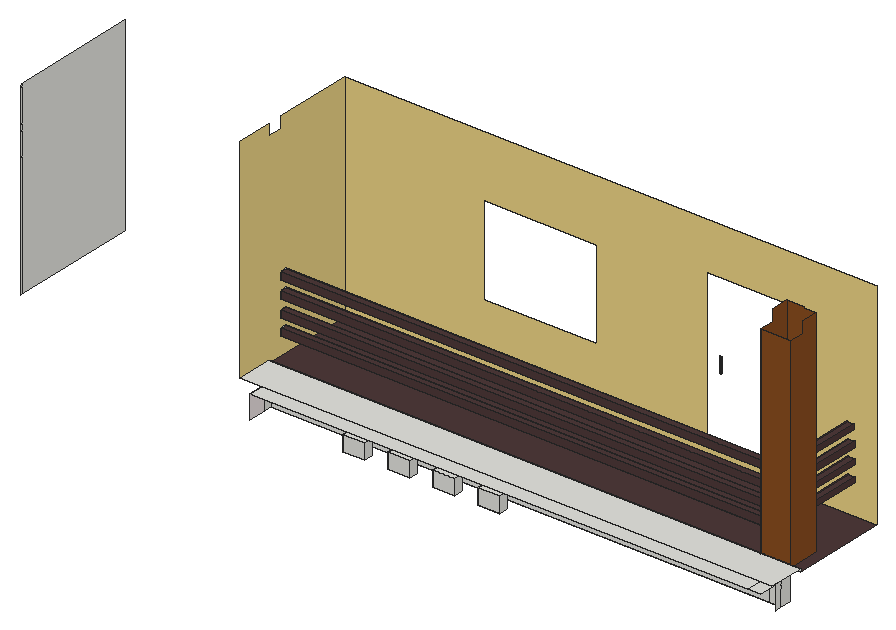
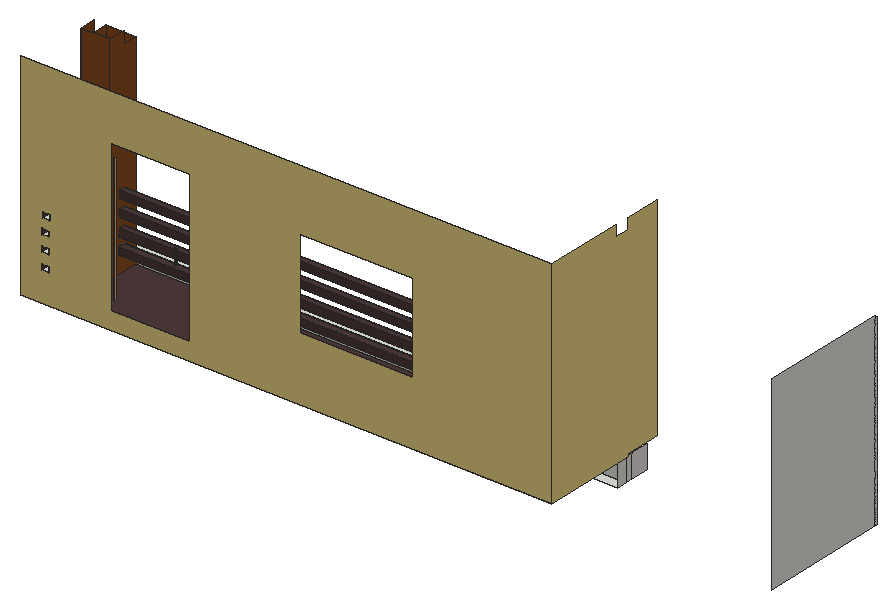
# SketchUp Ruby script. Lengths in inches.
U = 1.inch
M = Sketchup.active_model
def pt(a) = Geom::Point3d.new(a.map { |v| v * U })
def face(e, loops, mat)
  f = e.add_face(loops[0].map { |a| pt(a) })
  loops[1..].each { |l| e.add_face(l.map { |a| pt(a) }).erase! }
  f.material = f.back_material = mat if mat
  f
end
# faces: each face lists its corners as indices into pts; further lists are holes
def faces(e, pts, list, mat = nil) = list.each { |f| face(e, (f[0].is_a?(Array) ? f : [f]).map { |l| l.map { |i| pts[i] } }, mat) }
# xy, xz, yz: faces in a plane at the given z, y or x. An outline is a flat list of corners, or four numbers for a rectangle; further outlines are holes
def ring(l) = l.size == 4 ? [[l[0], l[1]], [l[2], l[1]], [l[2], l[3]], [l[0], l[3]]] : l.each_slice(2).to_a
def flat(e, list, mat, &to3) = list.each { |f| face(e, (f[0].is_a?(Array) ? f : [f]).map { |l| ring(l).map { |u, v| to3.(u, v) } }, mat) }
def xy(e, z, list, mat = nil) = flat(e, list, mat) { |x, y| [x, y, z] }
def xz(e, y, list, mat = nil) = flat(e, list, mat) { |x, z| [x, y, z] }
def yz(e, x, list, mat = nil) = flat(e, list, mat) { |y, z| [x, y, z] }
def lines(e, pts, list) = list.each { |a, b| e.add_line(pt(pts[a]), pt(pts[b])) }
# prism: a flat outline (further loops are holes) pulled along v
def prism(e, loops, v, mat = nil)
  f = face(e, loops, mat); d = Geom::Vector3d.new(v.map { |x| x * U })
  f.pushpull(f.normal.samedirection?(d) ? d.length : -d.length)
end
def box(e, o, s, mat = nil) = prism(e, [[o, [o[0] + s[0], o[1], o[2]], [o[0] + s[0], o[1] + s[1], o[2]], [o[0], o[1] + s[1], o[2]]]], [0, 0, s[2]], mat)
def at(x, y, z, deg = 0) = Geom::Transformation.translation(pt([x, y, z])) * Geom::Transformation.rotation(ORIGIN, Z_AXIS, deg.degrees)
def axes(o, x, y, z) = Geom::Transformation.new([*x, 0, *y, 0, *z, 0, *pt(o).to_a, 1])
def part(name) = M.definitions.add(name)
# library, detail: a bought-in or finely detailed component or shape, given as its bounding box
def library(name, o, s) = part(name).tap { |d| box(d.entities, o, s) }
def detail(e, o, s) = box(e.add_group.entities, o, s)
def put(e, d, t, mat = nil) = e.add_instance(d, t).tap { |i| i.material = mat if mat }
def group(e, t, mat = nil) = e.add_group.tap { |g| g.transformation = t; g.material = mat if mat }.entities
root = M.entities
M.materials.add("Generic").color = [136, 77, 32]
M.materials.add("Generic\#2").color = [78, 57, 57]
M.materials.add("Generic\#3").color = [235, 210, 133]
M.materials.add("Generic\#5").color = [232, 222, 222]
M.materials.add("Material \#1").color = [140, 140, 140]
c1 = library("3DGeom~9_Defintion",[456.52,-471.89,-18.89],[5.57,1000,5.49])
xy(root,122.7629,[[180.7096,46.9375,193.0221,51.9375],[205.9596,46.9375,218.2721,51.9375],[231.2096,46.9375,243.5221,51.9375],[256.4596,46.9375,268.7721,51.9375]])
xy(root,131.3879,[[180.7096,46.9375,193.0221,51.9375],[205.9596,46.9375,218.2721,51.9375],[231.2096,46.9375,243.5221,51.9375],[256.4596,46.9375,268.7721,51.9375]])
xy(root,137.6106,[[411.67,41.4375,418.8848,51.9375],[411.67,51.9375,418.8848,55.875]])
xy(root,141.9375,[[412.79,61.6875,419.4775,79.5282]])
xy(root,141.9375,[[127.5829,61.6875,127.5829,114.8125,424.8848,114.8125,424.8848,61.6875,419.4775,61.6875,419.4775,79.5282,402.9775,79.5282,402.9775,61.6875]],"Generic\#2")
xy(root,143.5,[[127.5829,41.4375,424.8848,61.6875]])
xy(root,158.7077,[[409.2127,79.5282,412.7127,114.8126]])
xy(root,161.8952,[[409.2127,79.5282,412.7127,114.8126]],"Generic\#2")
xy(root,167.7702,[[409.2127,79.5282,412.7127,114.8126]])
xy(root,170.9577,[[409.2127,79.5282,412.7127,114.8126]],"Generic\#2")
xy(root,176.5202,[[409.2127,79.5282,412.7127,114.8126]])
xy(root,179.7077,[[409.2127,79.5282,412.7127,114.8126]],"Generic\#2")
xy(root,184.9607,[[408.521,79.5282,412.021,114.8126]])
xy(root,188.1482,[[408.521,79.5282,412.021,114.8126]],"Generic\#2")
xy(root,190.2391,[[338.0444,114.5846,338.0444,114.9056,338.0796,114.9056],[338.0444,114.5846,338.0796,114.9056,338.0796,114.5846]],"Material \#1")
xy(root,190.5551,[[338.0267,114.5846,338.0855,114.5846,338.0267,114.9056],[338.0855,114.5846,338.0855,114.9056,338.0267,114.9056]],"Material \#1")
xz(root,46.9375,[[180.7096,122.7629,193.0221,131.3879],[205.9596,122.7629,218.2721,131.3879],[231.2096,122.7629,243.5221,131.3879],[256.4596,122.7629,268.7721,131.3879]])
xz(root,55.875,[[411.67,124.5524,411.67,137.6106,133.3329,137.6107,133.334,124.5525],[411.67,124.5524,418.8844,124.5524,418.8848,137.6106,411.67,137.6106]])
xz(root,61.6875,[[127.5829,141.9375,402.9775,143.5],[402.9775,141.9375,412.79,143.5],[412.79,141.9375,419.4775,143.5],[419.4775,141.9375,424.8848,143.5]])
xz(root,61.6875,[[402.9775,143.5,419.4775,255.6875]],"Generic")
xz(root,69.8538,[[127.5793,151.8312,402.9775,155.8937],[127.5793,160.9562,402.9775,165.0187],[127.5793,170.6437,402.9775,174.7062],[127.5793,180.1437,402.9775,184.2062]],"Generic\#2")
xz(root,73.6426,[[127.5793,151.8384,402.9775,155.9009],[127.5793,160.9634,402.9775,165.0259],[127.5793,170.6509,402.9775,174.7134],[127.5793,180.1509,402.9775,184.2134]],"Generic\#2")
xz(root,79.5282,[[409.2127,158.7077,412.7127,161.8952],[409.2127,167.7702,412.7127,170.9577],[409.2127,176.5202,412.7127,179.7077],[408.521,184.9607,412.021,188.1482]])
xz(root,79.5282,[[[402.9775,141.9375,419.4775,141.9375,419.4775,261.9375,412.79,261.9375,412.79,262.375,402.9775,262.375],[408.521,184.9607,412.021,188.1482],[409.2127,176.5202,412.7127,179.7077],[409.2127,167.7702,412.7127,170.9577],[409.2127,158.7077,412.7127,161.8952]]],"Generic")
xz(root,114.5846,[[338.0558,190.1859,337.9996,190.1931,338.0558,190.1938],[338.0558,190.1859,338.0558,190.1938,338.1099,190.2008],[338.0558,190.1859,338.1099,190.2008,338.1121,190.1931],[337.9996,190.1931,337.9472,190.2142,338.0017,190.2008],[337.9996,190.1931,338.0017,190.2008,338.0558,190.1938],
  [338.1121,190.1931,338.1099,190.2008,338.1603,190.2211],[338.1121,190.1931,338.1603,190.2211,338.1644,190.2142],[338.0017,190.2008,337.9472,190.2142,337.9513,190.2211],[337.9472,190.2142,337.9023,190.2477,337.9513,190.2211],[338.1644,190.2142,338.1603,190.2211,338.2036,190.2534],
  [338.1644,190.2142,338.2036,190.2534,338.2094,190.2477],[337.9513,190.2211,337.9023,190.2477,337.9081,190.2534],[337.9023,190.2477,337.8677,190.2915,337.9081,190.2534],[338.2094,190.2477,338.2036,190.2534,338.2369,190.2955],[338.2094,190.2477,338.2369,190.2955,338.2439,190.2915],
  [337.9081,190.2534,337.8677,190.2915,337.8748,190.2955],[337.8677,190.2915,337.846,190.3424,337.8748,190.2955],[338.2439,190.2915,338.2369,190.2955,338.2577,190.3445],[338.2439,190.2915,338.2577,190.3445,338.2656,190.3424],[337.8748,190.2955,337.846,190.3424,337.854,190.3445],
  [337.846,190.3424,337.8386,190.3971,337.854,190.3445],[338.2656,190.3424,338.2577,190.3445,338.2649,190.3971],[338.2656,190.3424,338.2649,190.3971,338.273,190.3971],[337.854,190.3445,337.8386,190.3971,337.8468,190.3971],[337.8386,190.3971,337.846,190.4517,337.8468,190.3971],
  [337.8468,190.3971,337.846,190.4517,337.854,190.4497],[338.2649,190.3971,338.2577,190.4497,338.273,190.3971],[338.273,190.3971,338.2577,190.4497,338.2656,190.4517],[337.854,190.4497,337.846,190.4517,337.8677,190.5027],[337.854,190.4497,337.8677,190.5027,337.8748,190.4987],
  [338.2577,190.4497,338.2369,190.4987,338.2656,190.4517],[338.2656,190.4517,338.2369,190.4987,338.2439,190.5027],[337.8748,190.4987,337.8677,190.5027,337.9023,190.5464],[337.8748,190.4987,337.9023,190.5464,337.9081,190.5408],[338.2369,190.4987,338.2036,190.5408,338.2439,190.5027],
  [338.2439,190.5027,338.2036,190.5408,338.2094,190.5464],[337.9081,190.5408,337.9023,190.5464,337.9472,190.58],[337.9081,190.5408,337.9472,190.58,337.9513,190.5731],[338.2036,190.5408,338.1603,190.5731,338.2094,190.5464],[338.2094,190.5464,338.1603,190.5731,338.1644,190.58],
  [337.9513,190.5731,337.9472,190.58,337.9996,190.6011],[337.9513,190.5731,337.9996,190.6011,338.0017,190.5934],[338.1603,190.5731,338.1099,190.5934,338.1644,190.58],[338.1644,190.58,338.1099,190.5934,338.1121,190.6011],[338.0017,190.5934,337.9996,190.6011,338.0558,190.6083],
  [338.0017,190.5934,338.0558,190.6083,338.0558,190.6003],[338.1099,190.5934,338.0558,190.6003,338.1121,190.6011],[338.0558,190.6003,338.0558,190.6083,338.1121,190.6011]],"Material \#1")
xz(root,114.595,[[338.0558,189.7138,337.9354,189.77,338.1763,189.77],[338.0558,189.7138,337.988,189.729,337.9354,189.77],[338.0558,189.7138,338.0205,189.7177,337.988,189.729],[338.0558,189.7138,338.1237,189.729,338.0912,189.7177],[338.0558,189.7138,338.1763,189.77,338.1237,189.729],
  [337.988,189.729,337.9593,189.7468,337.9354,189.77],[338.1237,189.729,338.1763,189.77,338.1523,189.7468],[338.1763,189.77,337.782,190.3616,337.8657,190.2489],[338.1763,189.77,337.8956,190.1739,337.782,190.3616],[338.1763,189.77,337.8657,190.2489,337.9035,190.2122],
  [338.1763,189.77,337.8982,190.1686,337.8956,190.1739],[338.1763,189.77,337.9,190.163,337.8982,190.1686],[338.1763,189.77,337.9011,190.1571,337.9,190.163],[337.9354,189.77,337.9011,190.1571,338.1763,189.77],[337.9354,189.77,337.9015,190.151,337.9011,190.1571],
  [337.9354,189.77,337.9056,189.8295,337.9015,190.151],[338.1763,189.77,337.9035,190.2122,337.9487,190.1842],[337.9354,189.77,337.9172,189.7979,337.9056,189.8295],[338.1763,189.77,337.9487,190.1842,338,190.1664],[338.1763,189.77,338,190.1664,338.0558,190.1601],
  [338.1763,189.77,338.0558,190.1601,338.2102,189.8639],[338.1763,189.77,338.2061,189.8295,338.1945,189.7979],[338.1763,189.77,338.2102,189.8639,338.2061,189.8295],[337.9056,189.8295,337.9015,189.8639,337.9015,190.151],[338.2102,189.8639,338.0558,190.1601,338.1117,190.1664],
  [338.2102,189.8639,338.1117,190.1664,338.163,190.1842],[338.2102,189.8639,338.163,190.1842,338.2082,190.2122],[338.2102,189.8639,338.2082,190.2122,338.2102,190.151],[338.2102,190.151,338.2082,190.2122,338.2118,190.1636],[338.2102,190.151,338.2118,190.1636,338.2106,190.1576],
  [338.2118,190.1636,338.2082,190.2122,338.246,190.2489],[338.2118,190.1636,338.2165,190.1744,338.2137,190.1692],[338.2118,190.1636,338.246,190.2489,338.2165,190.1744],[337.8956,190.1739,337.8921,190.179,337.782,190.3616],[338.2165,190.1744,338.246,190.2489,338.2748,190.2929],
  [338.2165,190.1744,338.2748,190.2929,338.3295,190.3617],[338.2165,190.1744,338.3295,190.3617,338.2199,190.1792],[337.8921,190.179,337.8877,190.1839,337.782,190.3616],[338.2199,190.1792,338.3295,190.3617,338.2241,190.1839],[337.8877,190.1839,337.8346,190.2365,337.782,190.3616],
  [337.8877,190.1839,337.8825,190.1885,337.8346,190.2365],[338.2241,190.1839,338.2761,190.2374,338.229,190.1883],[338.2241,190.1839,338.3295,190.3617,338.2761,190.2374],[338.229,190.1883,338.2761,190.2374,338.2539,190.2116],[337.8825,190.1885,337.857,190.2111,337.8346,190.2365],
  [337.8346,190.2365,337.8004,190.295,337.782,190.3616],[337.8346,190.2365,337.8156,190.2646,337.8004,190.295],[338.2761,190.2374,338.3107,190.2957,338.2952,190.2655],[338.2761,190.2374,338.3295,190.3617,338.3107,190.2957],[337.8657,190.2489,337.782,190.3616,337.8369,190.2929],
  [337.8369,190.2929,337.782,190.3616,337.8186,190.3428],[338.2748,190.2929,338.2931,190.3428,338.3295,190.3617],[337.8004,190.295,337.789,190.3274,337.782,190.3616],[338.3107,190.2957,338.3295,190.3617,338.3223,190.3278],[337.8186,190.3428,337.782,190.3616,337.8121,190.3971],
  [338.2931,190.3428,338.2995,190.3971,338.3295,190.3617],[337.782,190.3616,337.7796,190.3971,337.7869,190.4586],[337.782,190.3616,337.7869,190.4586,337.8404,190.565],[337.782,190.3616,337.8186,190.4514,337.8121,190.3971],[337.782,190.3616,337.8404,190.565,337.8186,190.4514],
  [338.3295,190.3617,338.2713,190.565,338.3247,190.4586],[338.3295,190.3617,338.2748,190.5012,338.2713,190.565],[338.3295,190.3617,338.2931,190.4514,338.2748,190.5012],[338.3295,190.3617,338.2995,190.3971,338.2931,190.4514],[338.3295,190.3617,338.3247,190.4586,338.332,190.3971],
  [337.8186,190.4514,337.8404,190.565,337.8369,190.5012],[337.7869,190.4586,337.8077,190.5151,337.8404,190.565],[338.3247,190.4586,338.2713,190.565,338.3039,190.5151],[337.8369,190.5012,337.8404,190.565,337.8657,190.5453],[338.2748,190.5012,338.246,190.5453,338.2713,190.565],
  [337.8657,190.5453,337.8404,190.565,337.9035,190.582],[338.246,190.5453,338.2082,190.582,338.2713,190.565],[337.8404,190.565,337.8832,190.6066,337.9344,190.6383],[337.8404,190.565,337.9344,190.6383,338.0558,190.6657],[337.8404,190.565,337.9487,190.61,337.9035,190.582],
  [337.8404,190.565,338.0558,190.6657,337.9487,190.61],[338.2713,190.565,338.0558,190.6657,338.1772,190.6383],[338.2713,190.565,338.163,190.61,338.0558,190.6657],[338.2713,190.565,338.2082,190.582,338.163,190.61],[338.2713,190.565,338.1772,190.6383,338.2285,190.6066],
  [337.9487,190.61,338.0558,190.6657,338,190.6278],[338.163,190.61,338.1117,190.6278,338.0558,190.6657],[338,190.6278,338.0558,190.6657,338.0558,190.6341],[338.1117,190.6278,338.0558,190.6341,338.0558,190.6657],[337.9344,190.6383,337.9926,190.6586,338.0558,190.6657],
  [338.1772,190.6383,338.0558,190.6657,338.1191,190.6586]],"Material \#1")
xz(root,114.6295,[[338.0558,187.3364,337.9281,187.3476,338.0558,187.3483],[338.0558,187.3364,338.0558,187.3483,338.1814,187.3593],[338.0558,187.3364,338.1814,187.3593,338.1836,187.3476],[337.9281,187.3476,337.8081,187.3796,337.9303,187.3593],[337.9281,187.3476,337.9303,187.3593,338.0558,187.3483],
  [338.1836,187.3476,338.1814,187.3593,338.2993,187.3908],[338.1836,187.3476,338.2993,187.3908,338.3036,187.3796],[337.9303,187.3593,337.8081,187.3796,337.8123,187.3908],[337.8081,187.3796,337.6975,187.4307,337.8123,187.3908],[338.3036,187.3796,338.2993,187.3908,338.408,187.441],
  [338.3036,187.3796,338.408,187.441,338.4142,187.4307],[337.8123,187.3908,337.6975,187.4307,337.7037,187.441],[337.6975,187.4307,337.5983,187.499,337.7037,187.441],[338.4142,187.4307,338.408,187.441,338.5055,187.508],[338.4142,187.4307,338.5055,187.508,338.5134,187.499],
  [337.7037,187.441,337.5983,187.499,337.6062,187.508],[337.5983,187.499,337.5126,187.5823,337.6062,187.508],[338.5134,187.499,338.5055,187.508,338.5897,187.59],[338.5134,187.499,338.5897,187.59,338.5991,187.5823],[337.6062,187.508,337.5126,187.5823,337.5219,187.59],
  [338.0558,187.5212,338.0136,187.5249,338.0558,187.5331],[338.0558,187.5212,338.0558,187.5331,338.0959,187.5366],[338.0558,187.5212,338.0959,187.5366,338.0981,187.5249],[338.0136,187.5249,337.9736,187.5356,338.0158,187.5366],[338.0136,187.5249,338.0158,187.5366,338.0558,187.5331],
  [338.0981,187.5249,338.0959,187.5366,338.1339,187.5468],[338.0981,187.5249,338.1339,187.5468,338.1381,187.5356],[337.9736,187.5356,337.9367,187.5526,337.9778,187.5468],[337.9736,187.5356,337.9778,187.5468,338.0158,187.5366],[338.1381,187.5356,338.1339,187.5468,338.1688,187.5629],
  [338.1381,187.5356,338.1688,187.5629,338.175,187.5526],[337.9778,187.5468,337.9367,187.5526,337.9429,187.5629],[337.9367,187.5526,337.9038,187.5753,337.9429,187.5629],[338.175,187.5526,338.1688,187.5629,338.2,187.5844],[338.175,187.5526,338.2,187.5844,338.2079,187.5753],
  [337.9429,187.5629,337.9038,187.5753,337.9117,187.5844],[337.9038,187.5753,337.8754,187.6029,337.9117,187.5844],[338.2079,187.5753,338.2,187.5844,338.2269,187.6105],[338.2079,187.5753,338.2269,187.6105,338.2363,187.6029],[337.5126,187.5823,337.446,187.6728,337.5219,187.59],
  [338.5991,187.5823,338.5897,187.59,338.6587,187.6848],[338.5991,187.5823,338.6587,187.6848,338.6692,187.6788],[337.9117,187.5844,337.8754,187.6029,337.8848,187.6105],[337.5219,187.59,337.446,187.6728,337.4566,187.6789],[337.8754,187.6029,337.8521,187.6349,337.8848,187.6105],
  [338.2363,187.6029,338.2269,187.6105,338.249,187.6409],[338.2363,187.6029,338.249,187.6409,338.2596,187.6349],[337.8848,187.6105,337.8521,187.6349,337.8627,187.6409],[337.8521,187.6349,337.8346,187.6707,337.8627,187.6409],[338.2596,187.6349,338.249,187.6409,338.2656,187.6749],
  [338.2596,187.6349,338.2656,187.6749,338.2771,187.6707],[337.8627,187.6409,337.8346,187.6707,337.8461,187.6749],[337.8346,187.6707,337.8236,187.7096,337.8461,187.6749],[338.2771,187.6707,338.2656,187.6749,338.2761,187.7118],[338.2771,187.6707,338.2761,187.7118,338.2881,187.7097],
  [337.446,187.6728,337.3899,187.7863,337.4566,187.6789],[337.8461,187.6749,337.8236,187.7096,337.8356,187.7118],[338.6692,187.6788,338.6587,187.6848,338.7103,187.7904],[338.6692,187.6788,338.7103,187.7904,338.7218,187.7863],[337.4566,187.6789,337.3899,187.7863,337.4014,187.7905],
  [337.8236,187.7096,337.8198,187.7467,337.8356,187.7118],[338.2881,187.7097,338.2761,187.7118,338.2796,187.7507],[338.2881,187.7097,338.2796,187.7507,338.2919,187.7507],[337.8356,187.7118,337.8198,187.7467,337.832,187.7468],[337.8198,187.7467,337.8236,187.7917,337.832,187.7468],
  [337.832,187.7468,337.8236,187.7917,337.8356,187.7897],[338.2796,187.7507,338.2761,187.7897,338.2919,187.7507],[338.2919,187.7507,338.2761,187.7897,338.2881,187.7918],[337.3899,187.7863,337.3569,187.903,337.4014,187.7905],[338.7218,187.7863,338.7103,187.7904,338.7427,187.9051],
  [338.7218,187.7863,338.7427,187.9051,338.7548,187.903],[337.8356,187.7897,337.8236,187.7917,337.8346,187.8308],[337.8356,187.7897,337.8346,187.8308,337.8461,187.8266],[338.2761,187.7897,338.2656,187.8266,338.2881,187.7918],[337.4014,187.7905,337.3569,187.903,337.369,187.9051],
  [338.2881,187.7918,338.2656,187.8266,338.2771,187.8308],[337.8461,187.8266,337.8346,187.8308,337.8521,187.8666],[337.8461,187.8266,337.8521,187.8666,337.8627,187.8606],[338.2656,187.8266,338.249,187.8606,338.2771,187.8308],[338.2771,187.8308,338.249,187.8606,338.2596,187.8666],
  [337.8627,187.8606,337.8521,187.8666,337.8754,187.8986],[337.8627,187.8606,337.8754,187.8986,337.8848,187.8909],[338.249,187.8606,338.2269,187.8909,338.2596,187.8666],[338.2596,187.8666,338.2269,187.8909,338.2363,187.8986],[337.8848,187.8909,337.8754,187.8986,337.9038,187.9262],
  [337.8848,187.8909,337.9038,187.9262,337.9117,187.9171],[338.2269,187.8909,338.2,187.9171,338.2363,187.8986],[338.2363,187.8986,338.2,187.9171,338.2079,187.9262],[337.3569,187.903,337.345,188.0316,337.369,187.9051],[338.7548,187.903,338.7427,187.9051,338.7545,188.0322],
  [338.7548,187.903,338.7545,188.0322,338.7666,188.0316],[337.369,187.9051,337.345,188.0316,337.3572,188.0322],[337.9117,187.9171,337.9038,187.9262,337.9367,187.9488],[337.9117,187.9171,337.9367,187.9488,337.9429,187.9386],[338.2,187.9171,338.1688,187.9386,338.2079,187.9262],
  [338.2079,187.9262,338.1688,187.9386,338.175,187.9488],[337.9429,187.9386,337.9367,187.9488,337.9736,187.9659],[337.9429,187.9386,337.9736,187.9659,337.9778,187.9547],[338.1688,187.9386,338.1339,187.9547,338.175,187.9488],[338.175,187.9488,338.1339,187.9547,338.1381,187.9659],
  [337.9778,187.9547,337.9736,187.9659,338.0136,187.9766],[337.9778,187.9547,338.0136,187.9766,338.0158,187.9649],[338.1339,187.9547,338.0959,187.9649,338.1381,187.9659],[338.0158,187.9649,338.0136,187.9766,338.0558,187.9803],[338.0158,187.9649,338.0558,187.9803,338.0558,187.9684],
  [338.0959,187.9649,338.0558,187.9684,338.0981,187.9766],[338.0959,187.9649,338.0981,187.9766,338.1381,187.9659],[338.0558,187.9684,338.0558,187.9803,338.0981,187.9766],[337.345,188.0316,337.345,195.9223,337.3572,188.0322],[338.7666,188.0316,338.7545,188.0322,338.7545,194.2213],
  [338.7666,188.0316,338.7545,194.2213,338.7545,195.9218],[338.7666,188.0316,338.7545,195.9218,338.7666,195.9223],[337.3572,188.0322,337.345,195.9223,337.3572,195.9218]],"Material \#1")
xz(root,114.664,[[338.0558,190.1601,337.9928,190.1682,338.0558,190.1681],[338.0558,190.1601,338.0558,190.1681,338.1168,190.1759],[338.0558,190.1601,338.1168,190.1759,338.1189,190.1682],[338.0558,190.1681,337.9928,190.1682,337.9949,190.1759],[337.9928,190.1682,337.934,190.1918,337.9949,190.1759],
  [338.1189,190.1682,338.1168,190.1759,338.1736,190.1987],[338.1189,190.1682,338.1736,190.1987,338.1777,190.1918],[337.9949,190.1759,337.934,190.1918,337.9381,190.1987],[337.934,190.1918,337.8835,190.2295,337.9381,190.1987],[338.1777,190.1918,338.1736,190.1987,338.2224,190.2351],
  [338.1777,190.1918,338.2224,190.2351,338.2282,190.2295],[337.9381,190.1987,337.8835,190.2295,337.8893,190.2351],[337.8835,190.2295,337.8448,190.2786,337.8893,190.2351],[338.2282,190.2295,338.2224,190.2351,338.2598,190.2826],[338.2282,190.2295,338.2598,190.2826,338.2669,190.2786],
  [337.8893,190.2351,337.8448,190.2786,337.8519,190.2826],[337.8448,190.2786,337.8204,190.3357,337.8519,190.2826],[338.2669,190.2786,338.2598,190.2826,338.2833,190.3378],[338.2669,190.2786,338.2833,190.3378,338.2912,190.3357],[337.8519,190.2826,337.8204,190.3357,337.8284,190.3378],
  [337.8204,190.3357,337.8121,190.3971,337.8284,190.3378],[338.2912,190.3357,338.2833,190.3378,338.2914,190.3971],[338.2912,190.3357,338.2914,190.3971,338.2995,190.3971],[337.8284,190.3378,337.8121,190.3971,337.8203,190.3971],[337.8121,190.3971,337.8204,190.4584,337.8203,190.3971],
  [337.8203,190.3971,337.8204,190.4584,337.8284,190.4564],[338.2914,190.3971,338.2833,190.4564,338.2995,190.3971],[338.2995,190.3971,338.2833,190.4564,338.2912,190.4584],[337.8284,190.4564,337.8204,190.4584,337.8448,190.5156],[337.8284,190.4564,337.8448,190.5156,337.8519,190.5116],
  [338.2833,190.4564,338.2598,190.5116,338.2912,190.4584],[338.2912,190.4584,338.2598,190.5116,338.2669,190.5156],[337.8519,190.5116,337.8448,190.5156,337.8835,190.5647],[337.8519,190.5116,337.8835,190.5647,337.8893,190.559],[338.2598,190.5116,338.2224,190.559,338.2669,190.5156],
  [338.2669,190.5156,338.2224,190.559,338.2282,190.5647],[337.8893,190.559,337.8835,190.5647,337.934,190.6023],[337.8893,190.559,337.934,190.6023,337.9381,190.5954],[338.2224,190.559,338.1736,190.5954,338.2282,190.5647],[338.2282,190.5647,338.1736,190.5954,338.1777,190.6023],
  [337.9381,190.5954,337.934,190.6023,337.9928,190.626],[337.9381,190.5954,337.9928,190.626,337.9949,190.6183],[338.1736,190.5954,338.1168,190.6183,338.1777,190.6023],[338.1777,190.6023,338.1168,190.6183,338.1189,190.626],[337.9949,190.6183,337.9928,190.626,338.0558,190.6341],
  [337.9949,190.6183,338.0558,190.6341,338.0558,190.6261],[338.1168,190.6183,338.0558,190.6261,338.1189,190.626],[338.1189,190.626,338.0558,190.6261,338.0558,190.6341]],"Material \#1")
xz(root,114.8125,[[4.8848,141.9375,4.892,141.9375,4.8848,247.422]])
xz(root,114.9056,[[338.0444,190.2391,338.0326,190.2628,338.0679,190.2628],[338.0444,190.2391,338.0679,190.2628,338.0796,190.2391],[338.0326,190.2628,338.0264,190.2707,338.0741,190.2707],[338.0326,190.2628,338.0741,190.2707,338.0679,190.2628],[338.0264,190.2707,338.0264,190.2884,338.0741,190.2884],
  [338.0264,190.2707,338.0741,190.2884,338.0741,190.2707],[338.0264,190.2884,338.0326,190.2964,338.0679,190.2964],[338.0264,190.2884,338.0679,190.2964,338.0741,190.2884],[338.0326,190.2964,338.0326,190.326,338.0796,190.326],[338.0326,190.2964,338.0796,190.326,338.0679,190.2964],
  [338.0326,190.326,338.0326,190.3536,338.0796,190.3536],[338.0326,190.326,338.0796,190.3536,338.0796,190.326],[338.0326,190.3536,338.0237,190.376,338.0886,190.376],[338.0326,190.3536,338.0886,190.376,338.0796,190.3536],[338.0237,190.376,338.0237,190.3984,338.0886,190.3984],
  [338.0237,190.376,338.0886,190.3984,338.0886,190.376],[338.0237,190.3984,338.0326,190.4208,338.0796,190.4208],[338.0237,190.3984,338.0796,190.4208,338.0886,190.3984],[338.0326,190.4208,338.0267,190.4366,338.0855,190.4366],[338.0326,190.4208,338.0855,190.4366,338.0796,190.4208],
  [338.0267,190.4366,338.0267,190.4879,338.0855,190.4879],[338.0267,190.4366,338.0855,190.4879,338.0855,190.4366],[338.0267,190.4879,338.0339,190.4919,338.0783,190.4919],[338.0267,190.4879,338.0783,190.4919,338.0855,190.4879],[338.0339,190.4919,338.0339,190.4998,338.0783,190.4998],
  [338.0339,190.4919,338.0783,190.4998,338.0783,190.4919],[338.0339,190.4998,338.0267,190.5037,338.0855,190.5037],[338.0339,190.4998,338.0855,190.5037,338.0783,190.4998],[338.0267,190.5037,338.0267,190.5551,338.0855,190.5551],[338.0267,190.5037,338.0855,190.5551,338.0855,190.5037]],"Material \#1")
xz(root,114.9401,[[338.0558,189.7138,337.988,189.729,338.0205,189.7177],[338.0558,189.7138,338.1237,189.729,337.988,189.729],[338.0558,189.7138,338.0912,189.7177,338.1237,189.729],[337.988,189.729,337.9015,190.151,337.9056,189.8295],[337.988,189.729,338.2061,189.8295,337.9015,190.151],
  [337.988,189.729,337.9056,189.8295,337.9354,189.77],[337.988,189.729,337.9354,189.77,337.9593,189.7468],[337.988,189.729,338.1237,189.729,338.2061,189.8295],[338.1237,189.729,338.1523,189.7468,338.1763,189.77],[338.1237,189.729,338.1763,189.77,338.2061,189.8295],
  [337.9354,189.77,337.9056,189.8295,337.9172,189.7979],[338.1763,189.77,338.1945,189.7979,338.2061,189.8295],[338.2061,189.8295,337.8956,190.1739,337.8982,190.1686],[338.2061,189.8295,338.2102,189.8639,337.8956,190.1739],[338.2061,189.8295,337.8982,190.1686,337.9,190.163],
  [338.2061,189.8295,337.9,190.163,337.9011,190.1571],[338.2061,189.8295,337.9011,190.1571,337.9015,190.151],[337.9056,189.8295,337.9015,190.151,337.9015,189.8639],[338.2102,189.8639,337.8657,190.2489,337.8956,190.1739],[338.2102,189.8639,337.9035,190.2122,337.8657,190.2489],
  [338.2102,189.8639,337.9487,190.1842,337.9035,190.2122],[338.2102,189.8639,338,190.1664,337.9487,190.1842],[338.2102,189.8639,338.0558,190.1601,338,190.1664],[338.2102,189.8639,338.1117,190.1664,338.0558,190.1601],[338.2102,189.8639,338.2102,190.151,338.1117,190.1664],
  [338.2102,190.151,338.2118,190.1636,338.1117,190.1664],[338.2102,190.151,338.2106,190.1576,338.2118,190.1636],[338.2118,190.1636,338.2165,190.1744,338.1117,190.1664],[338.2118,190.1636,338.2137,190.1692,338.2165,190.1744],[338.1117,190.1664,338.2165,190.1744,338.163,190.1842],
  [337.8956,190.1739,337.782,190.3616,337.8921,190.179],[337.8956,190.1739,337.8369,190.2929,337.782,190.3616],[337.8956,190.1739,337.8657,190.2489,337.8369,190.2929],[338.2165,190.1744,338.2082,190.2122,338.163,190.1842],[338.2165,190.1744,338.246,190.2489,338.2082,190.2122],
  [338.2165,190.1744,338.2199,190.1792,338.3295,190.3617],[338.2165,190.1744,338.3295,190.3617,338.246,190.2489],[337.8921,190.179,337.782,190.3616,337.8877,190.1839],[338.2199,190.1792,338.2241,190.1839,338.3295,190.3617],[337.8877,190.1839,337.782,190.3616,337.8346,190.2365],
  [337.8877,190.1839,337.8346,190.2365,337.8825,190.1885],[338.2241,190.1839,338.229,190.1883,338.2761,190.2374],[338.2241,190.1839,338.2761,190.2374,338.3295,190.3617],[338.229,190.1883,338.2539,190.2116,338.2761,190.2374],[337.8825,190.1885,337.8346,190.2365,337.857,190.2111],
  [337.8346,190.2365,337.782,190.3616,337.8004,190.295],[337.8346,190.2365,337.8004,190.295,337.8156,190.2646],[338.2761,190.2374,338.2952,190.2655,338.3107,190.2957],[338.2761,190.2374,338.3107,190.2957,338.3295,190.3617],[338.246,190.2489,338.3295,190.3617,338.2748,190.2929],
  [337.8369,190.2929,337.8186,190.3428,337.782,190.3616],[338.2748,190.2929,338.3295,190.3617,338.2931,190.3428],[337.8004,190.295,337.782,190.3616,337.789,190.3274],[338.3107,190.2957,338.3223,190.3278,338.3295,190.3617],[337.8186,190.3428,337.8121,190.3971,337.782,190.3616],
  [338.2931,190.3428,338.3295,190.3617,338.2995,190.3971],[337.782,190.3616,337.7869,190.4586,337.7796,190.3971],[337.782,190.3616,337.8121,190.3971,337.8186,190.4514],[337.782,190.3616,337.8186,190.4514,337.8369,190.5012],[337.782,190.3616,337.8369,190.5012,337.8404,190.565],
  [337.782,190.3616,337.8404,190.565,337.7869,190.4586],[338.3295,190.3617,338.2713,190.565,338.2931,190.4514],[338.3295,190.3617,338.3247,190.4586,338.2713,190.565],[338.3295,190.3617,338.2931,190.4514,338.2995,190.3971],[338.3295,190.3617,338.332,190.3971,338.3247,190.4586],
  [338.2931,190.4514,338.2713,190.565,338.2748,190.5012],[337.7869,190.4586,337.8404,190.565,337.8077,190.5151],[338.3247,190.4586,338.3039,190.5151,338.2713,190.565],[337.8369,190.5012,337.8657,190.5453,337.8404,190.565],[338.2748,190.5012,338.2713,190.565,338.246,190.5453],
  [337.8657,190.5453,337.9035,190.582,337.8404,190.565],[338.246,190.5453,338.2713,190.565,338.2082,190.582],[337.8404,190.565,337.9035,190.582,337.9487,190.61],[337.8404,190.565,337.9344,190.6383,337.8832,190.6066],[337.8404,190.565,337.9487,190.61,338.0558,190.6657],
  [337.8404,190.565,338.0558,190.6657,337.9344,190.6383],[338.2713,190.565,338.0558,190.6657,338.163,190.61],[338.2713,190.565,338.1772,190.6383,338.0558,190.6657],[338.2713,190.565,338.163,190.61,338.2082,190.582],[338.2713,190.565,338.2285,190.6066,338.1772,190.6383],
  [337.9487,190.61,338,190.6278,338.0558,190.6657],[338.163,190.61,338.0558,190.6657,338.1117,190.6278],[338,190.6278,338.0558,190.6341,338.0558,190.6657],[338.1117,190.6278,338.0558,190.6657,338.0558,190.6341],[337.9344,190.6383,338.0558,190.6657,337.9926,190.6586],
  [338.1772,190.6383,338.1191,190.6586,338.0558,190.6657]],"Material \#1")
yz(root,4.8848,[[41.4375,141.9375,42.5,246.5106],[42.5,141.9375,114.8125,247.422]])
yz(root,127.5793,[[69.8538,151.8312,69.8538,155.8937,73.6426,155.9009,73.6426,151.8384],[69.8538,160.9562,69.8538,165.0187,73.6426,165.0259,73.6426,160.9634],[69.8538,170.6437,69.8538,174.7062,73.6426,174.7134,73.6426,170.6509],[69.8538,180.1437,69.8538,184.2062,73.6426,184.2134,73.6426,180.1509]])
yz(root,180.7096,[[46.9375,122.7629,51.9375,131.3879]])
yz(root,193.0221,[[46.9375,122.7629,51.9375,131.3879]])
yz(root,205.9596,[[46.9375,122.7629,51.9375,131.3879]])
yz(root,218.2721,[[46.9375,122.7629,51.9375,131.3879]])
yz(root,231.2096,[[46.9375,122.7629,51.9375,131.3879]])
yz(root,243.5221,[[46.9375,122.7629,51.9375,131.3879]])
yz(root,256.4596,[[46.9375,122.7629,51.9375,131.3879]])
yz(root,268.7721,[[46.9375,122.7629,51.9375,131.3879]])
yz(root,338.0267,[[114.9056,190.5037,114.5846,190.5551,114.9056,190.5551]],"Material \#1")
yz(root,338.0326,[[114.9056,190.2964,114.5846,190.326,114.9056,190.326]],"Material \#1")
yz(root,338.0796,[[114.5846,190.326,114.9056,190.326,114.9056,190.3536],[114.5846,190.326,114.9056,190.3536,114.5846,190.3536]],"Material \#1")
yz(root,338.0855,[[114.5846,190.4366,114.9056,190.4366,114.9056,190.4879]],"Material \#1")
yz(root,338.0886,[[114.5846,190.376,114.9056,190.376,114.9056,190.3984],[114.5846,190.376,114.9056,190.3984,114.5846,190.3984]],"Material \#1")
yz(root,402.9775,[[69.8538,151.8312,73.6426,151.8384,73.6426,155.9009,69.8538,155.8937],[69.8538,160.9562,73.6426,160.9634,73.6426,165.0259,69.8538,165.0187],[69.8538,170.6437,73.6426,170.6509,73.6426,174.7134,69.8538,174.7062],[69.8538,180.1437,73.6426,180.1509,73.6426,184.2134,69.8538,184.2062]])
yz(root,402.9775,[[[61.6875,141.9375,79.5282,141.9375,79.5282,262.375,70.125,262.375,70.125,255.6875,61.6875,255.6875],[69.8538,180.1437,69.8538,184.2062,73.6426,184.2134,73.6426,180.1509],[69.8538,170.6437,69.8538,174.7062,73.6426,174.7134,73.6426,170.6509],[69.8538,160.9562,69.8538,165.0187,73.6426,165.0259,73.6426,160.9634],[69.8538,151.8312,69.8538,155.8937,73.6426,155.9009,73.6426,151.8384]]],"Generic")
yz(root,408.521,[[79.5282,184.9607,114.8126,188.1482]],"Generic\#2")
yz(root,409.2127,[[79.5282,158.7077,114.8126,161.8952],[79.5282,167.7702,114.8126,170.9577],[79.5282,176.5202,114.8126,179.7077]],"Generic\#2")
yz(root,412.021,[[79.5282,184.9607,114.8126,188.1482]],"Generic\#2")
yz(root,412.7127,[[79.5282,158.7077,114.8126,161.8952],[79.5282,167.7702,114.8126,170.9577],[79.5282,176.5202,114.8126,179.7077]],"Generic\#2")
yz(root,419.4775,[[61.6875,141.9375,79.5282,141.9375,79.5282,261.9375,70.125,261.9375,70.125,255.6875,61.6875,255.6875]],"Generic")
p = [[133.334,41.4375,124.5525],[133.334,51.9375,124.5525],[133.3329,51.9375,137.6107],[133.3329,41.4375,137.6107],[133.3329,55.875,137.6107],[133.334,55.875,124.5525],
  [418.8844,55.875,124.5524],[418.8844,51.9375,124.5524],[418.8848,51.9375,137.6106],[418.8848,55.875,137.6106],[133.334,61.6875,124.5525],[418.8844,61.6875,124.5524],
  [411.67,55.875,124.5524],[133.3329,61.6875,137.6107],[418.8848,61.6875,137.6106],[411.67,51.9375,137.6106],[411.67,41.4375,137.6106],[411.67,55.875,137.6106],
  [127.5747,41.4375,261.9375],[127.5829,41.4375,143.5],[127.5829,61.6875,143.5],[127.5829,61.6875,141.9375],[127.5829,114.8125,141.9375],[127.5747,114.8125,261.9375],
  [127.5747,70.125,261.9375],[127.5747,70.125,255.6875],[127.5747,61.6875,255.6875],[127.5747,61.6875,261.9375],[127.5747,42.5,261.9375],[424.8848,114.8125,141.9375],
  [424.8848,114.8125,261.9375],[330.35,114.8125,235.7164],[374.475,114.8125,235.7164],[374.475,114.8125,151.7789],[330.35,114.8125,151.7789],[205.199,114.8125,177.7828],
  [205.199,114.8125,227.5328],[268.449,114.8125,227.5328],[268.449,114.8125,177.7828],[408.521,114.8126,184.9607],[408.521,114.8126,188.1482],[412.021,114.8126,188.1482],
  [412.021,114.8126,184.9607],[409.2127,114.8126,176.5202],[409.2127,114.8126,179.7077],[412.7127,114.8126,179.7077],[412.7127,114.8126,176.5202],[409.2127,114.8126,167.7702],
  [409.2127,114.8126,170.9577],[412.7127,114.8126,170.9577],[412.7127,114.8126,167.7702],[409.2127,114.8126,158.7077],[409.2127,114.8126,161.8952],[412.7127,114.8126,161.8952],
  [412.7127,114.8126,158.7077],[402.9775,73.6426,151.8384],[402.9775,69.8538,151.8312],[127.5793,69.8538,151.8312],[127.5793,73.6426,151.8384],[402.9775,69.8538,155.8937],
  [402.9775,73.6426,155.9009],[127.5793,73.6426,155.9009],[127.5793,69.8538,155.8937],[402.9775,73.6426,160.9634],[402.9775,69.8538,160.9562],[127.5793,69.8538,160.9562],
  [127.5793,73.6426,160.9634],[402.9775,69.8538,165.0187],[402.9775,73.6426,165.0259],[127.5793,73.6426,165.0259],[127.5793,69.8538,165.0187],[402.9775,73.6426,170.6509],
  [402.9775,69.8538,170.6437],[127.5793,69.8538,170.6437],[127.5793,73.6426,170.6509],[402.9775,69.8538,174.7062],[402.9775,73.6426,174.7134],[127.5793,73.6426,174.7134],
  [127.5793,69.8538,174.7062],[402.9775,73.6426,180.1509],[402.9775,69.8538,180.1437],[127.5793,69.8538,180.1437],[127.5793,73.6426,180.1509],[402.9775,69.8538,184.2062],
  [402.9775,73.6426,184.2134],[127.5793,73.6426,184.2134],[127.5793,69.8538,184.2062],[337.9565,114.6367,187.6595],[337.9565,114.6643,187.6595],[337.977,114.6643,187.6413],
  [337.977,114.6367,187.6413],[338.0019,114.6643,187.6286],[338.0019,114.6367,187.6286],[338.0195,114.6566,187.6535],[338.0195,114.629,187.6535],[338.0764,114.6263,187.8258],
  [338.0764,114.6539,187.8258],[337.9904,114.6539,187.7063],[337.9904,114.6263,187.7063],[337.9743,114.6566,187.6842],[337.9743,114.629,187.6842],[338.0352,114.6539,187.6757],
  [338.0352,114.6263,187.6757],[338.1214,114.6539,187.7952],[338.1214,114.6263,187.7952],[338.1373,114.6566,187.8172],[338.1373,114.629,187.8172],[338.1553,114.6643,187.8418],
  [338.1553,114.6367,187.8418],[338.1347,114.6643,187.8602],[338.1347,114.6367,187.8602],[338.1101,114.6367,187.8727],[338.1101,114.6643,187.8727],[338.0922,114.6566,187.848],
  [338.0922,114.629,187.848],[338.0295,114.5846,190.2667],[338.0326,114.9056,190.2628],[338.0444,114.9056,190.2391],[338.0444,114.5846,190.2391],[338.0295,114.5846,190.2667],
  [338.0679,114.9056,190.2628],[338.071,114.5846,190.2667],[338.0796,114.5846,190.2391],[338.0796,114.5846,190.2391],[338.0796,114.9056,190.2391],[338.0679,114.9056,190.2628],
  [338.0326,114.9056,190.2964],[338.0295,114.5846,190.2924],[338.0326,114.5846,190.326],[338.0326,114.9056,190.326],[338.0326,114.5846,190.326],[338.0282,114.5846,190.3648],
  [338.0295,114.5846,190.2924],[338.0264,114.9056,190.2884],[338.0264,114.9056,190.2707],[338.0295,114.5846,190.2667],[338.0295,114.5846,190.2924],[338.0326,114.9056,190.2964],
  [338.0264,114.9056,190.2884],[338.0295,114.5846,190.2667],[338.0264,114.9056,190.2707],[338.0326,114.9056,190.2628],[338.0282,114.5846,190.3648],[338.0326,114.9056,190.3536],
  [338.0326,114.9056,190.326],[338.0796,114.9056,190.326],[338.0796,114.5846,190.326],[338.071,114.5846,190.2924],[338.071,114.5846,190.2667],[338.0741,114.9056,190.2707],
  [338.0741,114.9056,190.2884],[338.071,114.5846,190.2924],[338.071,114.5846,190.2924],[338.0679,114.9056,190.2964],[338.0796,114.9056,190.326],[338.071,114.5846,190.2924],
  [338.0741,114.9056,190.2884],[338.0679,114.9056,190.2964],[338.071,114.5846,190.2667],[338.0679,114.9056,190.2628],[338.0741,114.9056,190.2707],[338.0326,114.9056,190.3536],
  [338.0282,114.5846,190.3648],[338.0237,114.5846,190.3872],[338.0237,114.9056,190.376],[338.0237,114.5846,190.3872],[338.0282,114.5846,190.4096],[338.0267,114.9056,190.4366],
  [338.0269,114.5846,190.44],[338.0294,114.5846,190.4924],[338.0326,114.9056,190.4208],[338.0297,114.5846,190.4287],[338.0269,114.5846,190.44],[338.0237,114.9056,190.3984],
  [338.0282,114.5846,190.4096],[338.0297,114.5846,190.4287],[338.0237,114.5846,190.3872],[338.0237,114.9056,190.376],[338.0326,114.9056,190.3536],[338.0294,114.5846,190.4924],
  [338.0267,114.9056,190.4879],[338.0267,114.9056,190.4366],[338.0269,114.5846,190.44],[338.0267,114.9056,190.4366],[338.0326,114.9056,190.4208],[338.0297,114.5846,190.4287],
  [338.0326,114.9056,190.4208],[338.0237,114.9056,190.3984],[338.0282,114.5846,190.4096],[338.0237,114.9056,190.3984],[338.0237,114.9056,190.376],[338.0855,114.9056,190.4879],
  [338.0824,114.5846,190.4975],[338.0855,114.5846,190.4366],[338.0855,114.9056,190.4366],[338.0855,114.5846,190.4366],[338.0796,114.5846,190.4208],[338.0796,114.9056,190.4208],
  [338.0796,114.5846,190.4208],[338.0886,114.5846,190.3984],[338.0886,114.9056,190.376],[338.0886,114.5846,190.376],[338.0796,114.5846,190.3536],[338.0796,114.5846,190.4208],
  [338.0796,114.9056,190.4208],[338.0855,114.9056,190.4366],[338.0886,114.5846,190.3984],[338.0886,114.9056,190.3984],[338.0796,114.9056,190.4208],[338.0796,114.5846,190.3536],
  [338.0796,114.9056,190.3536],[338.0886,114.9056,190.376],[338.0267,114.9056,190.5037],[338.0294,114.5846,190.4924],[338.0267,114.5846,190.5551],[338.0294,114.5846,190.4924],
  [338.0339,114.9056,190.4998],[338.0339,114.9056,190.4919],[338.0294,114.5846,190.4924],[338.0267,114.9056,190.5037],[338.0294,114.5846,190.4924],[338.0267,114.9056,190.4879],
  [338.0855,114.9056,190.5551],[338.0855,114.5846,190.5551],[338.0824,114.5846,190.4975],[338.0824,114.5846,190.4975],[338.0855,114.9056,190.5037],[338.0855,114.9056,190.5551],
  [338.0824,114.5846,190.4975],[338.0855,114.9056,190.4879],[338.0783,114.9056,190.4919],[338.0824,114.5846,190.4975],[338.0783,114.9056,190.4998],[338.0855,114.9056,190.5037],
  [338.0824,114.5846,190.4975],[4.892,114.8125,141.9375],[4.9579,114.8125,141.9375],[402.9775,71.0664,182.5117],[127.5793,71.0664,182.5117],[402.9775,71.0664,172.7617],
  [127.5793,71.0664,172.7617],[402.9775,71.0664,163.0117],[127.5793,71.0664,163.0117],[402.9775,71.0664,153.6367],[127.5793,71.0664,153.6367],[410.8438,79.5282,186.8267],
  [410.8438,114.8126,186.8267],[410.8438,79.5282,178.0142],[410.8438,114.8126,178.0142],[410.8438,79.5282,169.2017],[410.8438,114.8126,169.2017],[410.8438,79.5282,160.3892],
  [410.8438,114.8126,160.3892],[411.67,51.9375,124.5524]]
faces(root,p,[[0,1,2,3]],"Generic\#5")
faces(root,p,[[4,2,1,5],[6,7,8,9],[10,11,6,12,5],[13,10,5,4],[11,14,9,6],[3,2,15,16],[2,15,17,4],[14,13,4,17,9],
  [55,56,57,58],[63,64,65,66],[71,72,73,74],[79,80,81,82]])
faces(root,p,[[18,19,20,21,22,23,24,25,26,27,28],[[22,29,30,23],[31,32,33,34],[35,36,37,38],[39,40,41,42],[43,44,45,46],[47,48,49,50],[51,52,53,54]]],"Generic\#3")
faces(root,p,[[59,60,61,62],[67,68,69,70],[75,76,77,78],[83,84,85,86]],"Generic\#2")
faces(root,p,[[87,88,89],[89,90,87],[90,89,91],[91,92,90],[92,91,93],[93,94,92],[95,96,97],[97,98,95],
  [98,97,99],[99,100,98],[100,99,88],[88,87,100],[94,93,101],[101,102,94],[102,101,103],[103,104,102],
  [104,103,105],[105,106,104],[106,105,107],[107,108,106],[108,107,109],[109,110,108],[111,112,113],[113,114,111],
  [114,113,96],[96,95,114],[110,109,112],[112,111,110],[115,116,117],[117,118,119],[120,121,122],[123,124,125],
  [126,127,128],[129,130,131],[132,133,134],[134,135,132],[136,137,138],[139,140,141],[142,143,144],[145,146,147],
  [148,149,150],[150,151,148],[152,153,154],[155,156,157],[158,159,160],[161,162,163],[164,165,166],[167,168,169],
  [170,171,172],[173,174,175],[176,177,178],[179,180,181],[182,183,184],[185,186,187],[188,189,190],[191,192,193],
  [194,195,196],[197,198,199],[200,201,202],[203,204,205],[206,207,208],[209,210,211],[212,213,214],[215,216,217],
  [218,219,216],[220,217,221],[222,223,224],[225,226,227],[228,229,230],[231,232,233],[234,230,232]],"Material \#1")
lines(root,p,[[235,236],[237,238],[239,240],[241,242],[243,244],[245,246],[247,248],[249,250],[251,252],[12,253]])
put(root,c1,axes([338.06,116.32,191.98],[0.07296,0,0],[0,0,0.07095],[0,0.06199,0]),"Material \#1")
